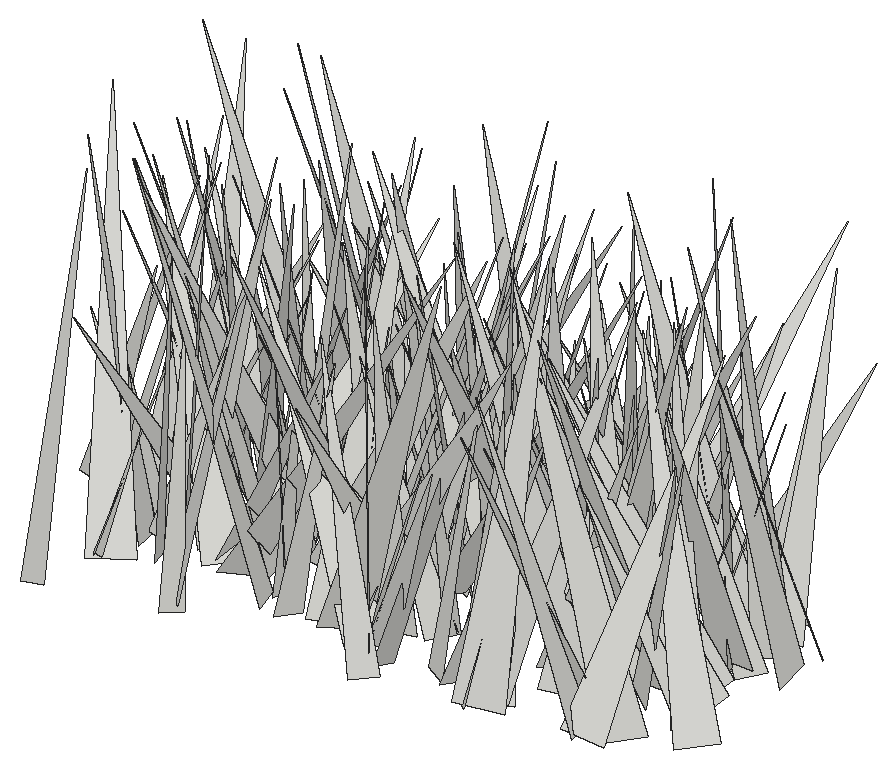
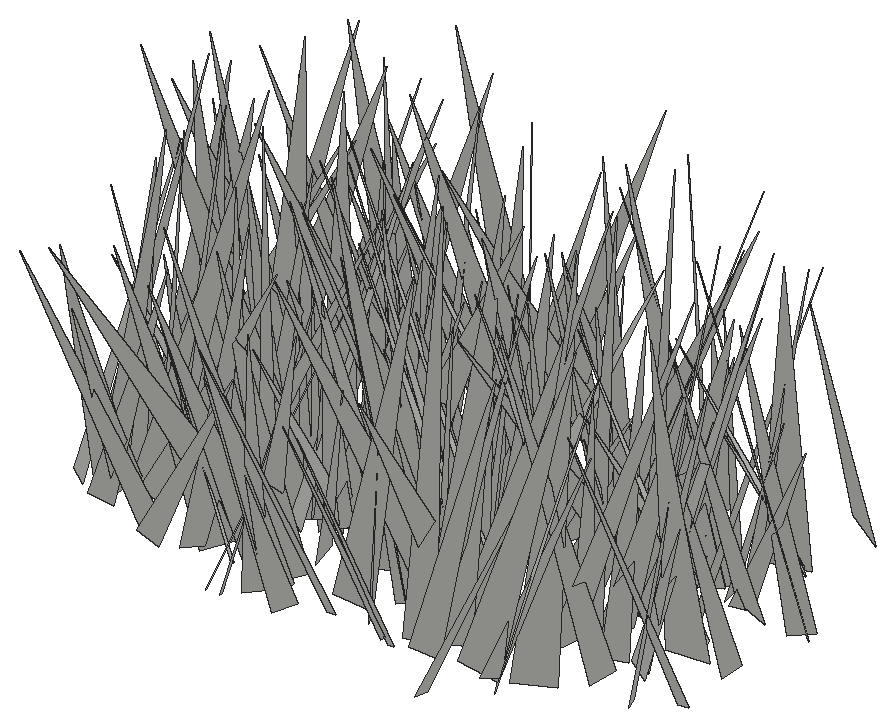
# SketchUp Ruby script. Lengths in inches.
U = 1.inch
M = Sketchup.active_model
def pt(a) = Geom::Point3d.new(a.map { |v| v * U })
def face(e, loops, mat)
  f = e.add_face(loops[0].map { |a| pt(a) })
  loops[1..].each { |l| e.add_face(l.map { |a| pt(a) }).erase! }
  f.material = f.back_material = mat if mat
  f
end
# faces: each face lists its corners as indices into pts; further lists are holes
def faces(e, pts, list, mat = nil) = list.each { |f| face(e, (f[0].is_a?(Array) ? f : [f]).map { |l| l.map { |i| pts[i] } }, mat) }
# xy, xz, yz: faces in a plane at the given z, y or x. An outline is a flat list of corners, or four numbers for a rectangle; further outlines are holes
def ring(l) = l.size == 4 ? [[l[0], l[1]], [l[2], l[1]], [l[2], l[3]], [l[0], l[3]]] : l.each_slice(2).to_a
def flat(e, list, mat, &to3) = list.each { |f| face(e, (f[0].is_a?(Array) ? f : [f]).map { |l| ring(l).map { |u, v| to3.(u, v) } }, mat) }
def xy(e, z, list, mat = nil) = flat(e, list, mat) { |x, y| [x, y, z] }
def xz(e, y, list, mat = nil) = flat(e, list, mat) { |x, z| [x, y, z] }
def yz(e, x, list, mat = nil) = flat(e, list, mat) { |y, z| [x, y, z] }
def lines(e, pts, list) = list.each { |a, b| e.add_line(pt(pts[a]), pt(pts[b])) }
# prism: a flat outline (further loops are holes) pulled along v
def prism(e, loops, v, mat = nil)
  f = face(e, loops, mat); d = Geom::Vector3d.new(v.map { |x| x * U })
  f.pushpull(f.normal.samedirection?(d) ? d.length : -d.length)
end
def box(e, o, s, mat = nil) = prism(e, [[o, [o[0] + s[0], o[1], o[2]], [o[0] + s[0], o[1] + s[1], o[2]], [o[0], o[1] + s[1], o[2]]]], [0, 0, s[2]], mat)
def at(x, y, z, deg = 0) = Geom::Transformation.translation(pt([x, y, z])) * Geom::Transformation.rotation(ORIGIN, Z_AXIS, deg.degrees)
def axes(o, x, y, z) = Geom::Transformation.new([*x, 0, *y, 0, *z, 0, *pt(o).to_a, 1])
def part(name) = M.definitions.add(name)
# library, detail: a bought-in or finely detailed component or shape, given as its bounding box
def library(name, o, s) = part(name).tap { |d| box(d.entities, o, s) }
def detail(e, o, s) = box(e.add_group.entities, o, s)
def put(e, d, t, mat = nil) = e.add_instance(d, t).tap { |i| i.material = mat if mat }
def group(e, t, mat = nil) = e.add_group.tap { |g| g.transformation = t; g.material = mat if mat }.entities
root = M.entities
c1 = part("fur_instance\#9")
p = [[0.8125,0,1.79],[0.67,-0.02,1.48],[0,-0.11,0],[0,0.11,0]]
faces(c1.entities,p,[[0,1,2,3]])
put(root,c1,axes([480.27,96.49,-21.66],[2.16067,6.65454,0.44246],[6.23565,-2.18071,2.34697],[-2.36543,0.32979,6.59114]))
put(root,c1,axes([500.39,100.44,-21.86],[-6.30832,-1.1114,1.05664],[-1.00602,6.37534,0.69964],[1.15742,-0.51611,6.36715]))
put(root,c1,axes([484.89,98.1,-21.86],[-4.63028,1.37895,0.71291],[1.15549,4.55932,-1.31404],[1.03661,1.07721,4.64912]))
put(root,c1,axes([491.26,100.58,-21.66],[3.99613,2.0991,0.80323],[2.24013,-3.58697,-1.77087],[0.18236,-1.93595,4.15203]))
put(root,c1,axes([500.77,100.9,-21.86],[-1.67937,-5.43767,0.87836],[-5.25266,1.30456,-1.96667],[-1.65811,1.37475,5.34049]))
put(root,c1,axes([492.84,98.29,-21.66],[-1.19348,5.65379,0.3473],[5.3271,0.99964,2.033],[-1.92561,-0.73875,5.40894]))
put(root,c1,axes([491.73,100.59,-21.86],[3.13596,-3.23192,0.2957],[-3.22644,-3.06024,0.76944],[0.35051,0.74607,4.43707]))
put(root,c1,axes([490.01,100.77,-21.86],[6.25642,-5.32962,1.03257],[-5.42827,-6.12142,1.29455],[0.06986,1.65444,8.11614]))
put(root,c1,axes([490.73,103.3,-21.86],[5.3138,-2.81187,1.14067],[-1.98861,-4.96443,-2.9739],[-2.29198,-2.2118,5.22484]))
put(root,c1,axes([496.16,99.26,-21.86],[2.60004,3.22909,0.64132],[3.22546,-2.66223,0.32783],[-0.65933,-0.2899,4.13277]))
put(root,c1,axes([490.37,102.97,-21.86],[-0.28332,-7.79704,0.77926],[-7.68212,0.12267,-1.56569],[-1.54472,0.82004,7.64347]))
put(root,c1,axes([491.24,100.57,-21.86],[4.97701,4.02381,2.97396],[4.34378,-5.5566,0.24873],[-2.48337,-1.65505,6.3953]))
put(root,c1,axes([486.82,100.67,-21.86],[-7.32124,-3.15954,0.71739],[-3.23761,7.2018,-1.32279],[0.12329,1.49974,7.86343]))
put(root,c1,axes([487.99,100.38,-21.86],[4.38322,-1.64948,1.59394],[-1.93146,-4.50849,0.64578],[-1.2373,1.19448,4.63858]))
put(root,c1,axes([496.82,99.37,-21.86],[-2.78975,7.45432,2.27613],[7.61508,3.12201,-0.8911],[1.66081,-1.79348,7.90921]))
put(root,c1,axes([497.34,100.01,-21.86],[-1.61358,3.38665,0.61033],[3.4322,1.63258,0.01498],[0.24881,-0.55751,3.75138]))
put(root,c1,axes([481.01,104.5,-21.86],[-5.2943,-3.28141,1.0592],[-2.29433,4.80125,3.40634],[2.57403,-2.46971,5.21479]))
put(root,c1,axes([494.33,100.22,-21.86],[2.52877,4.50107,1.40807],[4.66336,-2.62485,0.01569],[-0.70386,-1.21962,5.16276]))
put(root,c1,axes([494.9375,101.89,-21.86],[3.51068,-4.45404,1.06123],[-4.56743,-3.50052,0.41776],[-0.32136,1.09429,5.65587]))
put(root,c1,axes([491.55,101.67,-21.86],[1.40139,-5.88916,2.09043],[-6.21682,-1.53152,-0.14692],[-0.635,1.99706,6.05182]))
put(root,c1,axes([495.12,100.16,-21.86],[5.00649,-0.69371,1.01239],[-0.92226,-4.93206,1.18126],[-0.80969,1.32843,4.91435]))
put(root,c1,axes([491.03,100.64,-21.86],[-4.99082,4.3261,0.4502],[4.29852,4.80129,1.51542],[-0.66378,-1.43477,6.4286]))
put(root,c1,axes([484.51,98.6,-21.66],[4.61652,6.22378,1.13894],[6.03614,-4.75491,1.51682],[-1.89675,0.0163,7.59914]))
put(root,c1,axes([480.61,99.28,-21.66],[3.00596,2.69315,0.13963],[2.45938,-2.82346,1.51258],[-1.10635,1.04086,3.74179]))
put(root,c1,axes([487.03,101.47,-21.86],[-3.86454,-2.68359,1.87384],[-2.96857,4.09497,-0.25773],[1.3786,1.29506,4.69786]))
put(root,c1,axes([501.93,100.6875,-21.86],[-2.9065,7.574,1.65107],[7.44857,2.24028,2.83534],[-2.14716,-2.4809,7.60092]))
put(root,c1,axes([482.49,101.8,-21.86],[6.26613,3.81902,2.82967],[4.24719,-6.60086,-0.4964],[-2.13385,-1.92357,7.3214]))
put(root,c1,axes([482.27,100.73,-21.86],[-4.86729,-1.78674,2.25978],[-2.35287,5.02555,-1.09424],[1.66225,1.88173,5.06809]))
put(root,c1,axes([486.97,101.35,-21.86],[4.11345,0.18865,1.81103],[0.00918,-4.47631,0.44541],[-1.8208,0.4036,4.09361]))
put(root,c1,axes([481.49,101.72,-21.86],[0.33455,3.97904,1.71347],[4.11253,0.24873,-1.38056],[1.36232,-1.72801,3.74683]))
put(root,c1,axes([489.52,102.44,-21.66],[2.95462,-6.48005,1.02046],[-5.97059,-2.19282,3.36242],[2.71745,2.2277,6.27814]))
put(root,c1,axes([484.28,101.91,-21.86],[4.93305,-2.19664,0.15391],[-2.18894,-4.85066,0.92924],[0.23965,0.9109,5.31946]))
put(root,c1,axes([496.72,100.1875,-21.66],[1.72672,7.47142,1.23195],[7.48463,-1.49226,-1.44043],[1.14896,-1.50745,7.53186]))
put(root,c1,axes([481.16,101.46,-21.86],[-6.73527,-1.87686,1.53677],[-2.12146,6.75676,-1.04577],[1.17629,1.43931,6.91323]))
put(root,c1,axes([500.66,104.12,-21.86],[-0.93689,-7.58778,0.99671],[-7.63501,0.85799,-0.64504],[-0.52389,1.06539,7.61814]))
put(root,c1,axes([481.06,99.66,-21.86],[-3.36629,7.35026,0.38103],[7.33966,3.3212,0.77612],[-0.54849,-0.66835,8.0471]))
put(root,c1,axes([492.88,102.35,-21.86],[-3.29735,3.76242,1.32483],[3.9802,2.99017,1.41439],[-0.2628,-1.92005,4.79874]))
put(root,c1,axes([482,102.76,-21.66],[1.0853,-7.02468,2.48253],[-7.23303,-0.3918,2.05344],[1.78669,2.68091,6.80495]))
put(root,c1,axes([502.95,102.87,-21.86],[-4.62797,0.36048,0.06702],[0.36662,4.56134,0.78248],[0.00509,-0.78533,4.57556]))
put(root,c1,axes([500.76,102.97,-21.66],[-1.89095,-4.65132,2.366],[-4.60338,2.67208,1.57395],[2.45798,1.42605,4.76793]))
put(root,c1,axes([500.77,99.93,-21.86],[-1.75958,6.89289,0.89816],[6.66639,1.93582,-1.79628],[1.96924,-0.39424,6.88342]))
put(root,c1,axes([481.22,102.33,-21.86],[-3.86057,-0.50737,0.50019],[-0.53854,3.88252,-0.21837],[0.46646,0.28336,3.88764]))
put(root,c1,axes([486.08,102.13,-21.66],[-6.99068,-2.50094,0.47101],[-2.54423,6.83653,-1.46112],[-0.05835,1.53405,7.27938]))
put(root,c1,axes([492.55,99.67,-21.86],[7.12647,2.20024,1.82821],[1.44023,-6.99989,2.8102],[-2.47167,2.26505,6.90872]))
put(root,c1,axes([498.96,102.43,-21.86],[-8.06825,0.70999,0.37952],[0.71569,8.07597,0.10667],[0.36866,-0.13964,8.09873]))
put(root,c1,axes([477.54,103.22,-21.66],[1.22983,-5.08709,1.30795],[-5.046,-0.77126,1.74491],[1.45845,1.62123,4.93419]))
put(root,c1,axes([486.28,103.6875,-21.86],[-0.05824,-3.81958,0.55077],[-3.85535,0.08183,0.15984],[0.16986,0.54776,3.81668]))
put(root,c1,axes([485.17,101.18,-21.66],[7.21653,-2.33327,0.39687],[-2.31249,-6.67999,2.77668],[0.50399,2.75925,7.05779]))
put(root,c1,axes([494.375,103.38,-21.86],[7.07527,1.73735,2.55738],[2.12787,-7.36989,-0.88027],[-2.24293,-1.5114,7.23207]))
put(root,c1,axes([483.26,102.41,-21.86],[-3.33055,3.67395,0.98734],[3.8043,3.21801,0.85849],[0.0046,-1.30837,4.884]))
put(root,c1,axes([480.72,99.3,-21.66],[4.07419,5.57288,0.07978],[5.18286,-3.82462,2.48447],[-2.04971,1.40628,6.44076]))
put(root,c1,axes([484.37,101.42,-21.66],[-3.04335,5.85133,0.32291],[5.70958,2.87864,1.64877],[-1.32023,-1.03909,6.38604]))
put(root,c1,axes([480.43,102.84,-21.86],[-2.47066,2.78913,0.64805],[2.82871,2.24449,1.12431],[-0.44456,-1.21919,3.55237]))
put(root,c1,axes([499.96,104.59,-21.66],[5.73315,-1.08828,0.33068],[-0.98004,-5.58896,-1.40205],[-0.57725,-1.3198,5.66459]))
put(root,c1,axes([495.1,102.68,-21.86],[1.88047,-2.78184,1.95652],[-3.20631,-2.19563,-0.04014],[-1.13412,1.59479,3.35756]))
put(root,c1,axes([487.54,103.27,-21.66],[4.40599,-6.63506,1.39046],[-6.52465,-3.70025,3.01783],[1.84021,2.76664,7.37085]))
put(root,c1,axes([504.08,101.87,-21.86],[-4.84886,5.21937,0.60309],[5.25064,4.78392,0.8135],[-0.19034,-0.99462,7.07753]))
put(root,c1,axes([502.84,104.25,-21.86],[-6.49837,1.01991,0.13564],[1.01971,6.26851,1.71854],[-0.13717,-1.71841,6.34946]))
put(root,c1,axes([497.03,103.09,-21.86],[4.67154,-2.82363,0.84685],[-2.94301,-4.55853,1.0353],[-0.16964,1.32674,5.35951]))
put(root,c1,axes([485.5625,104.98,-21.86],[0.24896,-7.3468,1.55373],[-6.97419,-0.80255,-2.67734],[-2.78393,1.35351,6.84612]))
put(root,c1,axes([496.79,105.05,-21.86],[-0.95692,-4.60949,0.0097],[-4.59629,0.95343,-0.35816],[-0.34872,0.08227,4.69412]))
put(root,c1,axes([477.4,103.15,-21.66],[5.01329,4.55618,1.17415],[4.70331,-4.80639,-1.43108],[0.12753,-1.84671,6.62147]))
put(root,c1,axes([481.6,105.86,-21.86],[-5.06426,-4.56399,0.84014],[-4.29824,5.08189,1.69768],[1.74956,-0.72593,6.60262]))
put(root,c1,axes([494.05,106.69,-21.86],[1.8393,-7.94223,0.20343],[-7.82957,-1.84746,-1.33722],[-1.34842,-0.10629,8.04201]))
put(root,c1,axes([482.29,105.44,-21.86],[-3.33298,-6.74445,1.96036],[-6.484,3.7887,2.01069],[2.69971,0.77298,7.24938]))
put(root,c1,axes([491.25,105.73,-21.86],[-3.9717,-6.10655,1.7462],[-5.81347,4.32471,1.90107],[2.55787,0.34722,7.03209]))
put(root,c1,axes([499.71,103.1,-21.86],[-5.36752,5.77658,2.45123],[6.12108,5.53013,0.37117],[1.38195,-2.05828,7.87664]))
put(root,c1,axes([490.59,100.78,-21.66],[4.99959,5.18328,0.38062],[5.01525,-4.9501,1.53324],[-1.36326,0.79826,7.03643]))
put(root,c1,axes([490.82,103.55,-21.86],[-0.11529,-4.79427,2.44231],[-5.06003,0.9271,1.58106],[1.8292,2.26244,4.52754]))
put(root,c1,axes([498.22,101.44,-21.66],[-3.90191,2.21296,0.38649],[1.88444,3.64598,-1.85127],[1.22289,1.44261,4.08594]))
put(root,c1,axes([483.01,105.3125,-21.86],[7.66875,0.29762,1.40281],[0.64374,-7.5341,-1.92071],[-1.28143,-2.00373,7.43029]))
put(root,c1,axes([502.54,104.86,-21.66],[-6.59727,0.97904,0.29915],[1.02311,6.37288,1.70633],[0.03533,-1.73199,6.44755]))
put(root,c1,axes([493.36,102.35,-21.66],[-5.59441,-0.96055,0.72122],[-1.15543,5.24244,-1.98041],[0.32833,2.08191,5.31959]))
put(root,c1,axes([494.81,101.19,-21.86],[3.19327,6.60837,0.52108],[6.51338,-3.23542,1.11669],[-1.23207,0.02336,7.254]))
put(root,c1,axes([487.875,103.87,-21.86],[3.79573,2.84609,1.46317],[3.05532,-3.89817,-0.34352],[-0.95191,-1.16307,4.73179]))
put(root,c1,axes([503.25,102.5,-21.86],[-0.8728,6.82324,1.17968],[6.78553,0.6058,1.51645],[-1.38016,-1.33658,6.7096]))
put(root,c1,axes([501.84,106.55,-21.86],[2.0561,-6.44135,0.2848],[-6.4395,-2.06652,-0.24899],[-0.32395,0.19535,6.75697]))
put(root,c1,axes([498.01,104.34,-21.86],[7.40162,-2.04644,1.37858],[-2.14984,-7.48787,0.42713],[-1.21103,0.78507,7.66743]))
put(root,c1,axes([493.25,106.45,-21.86],[0.94954,-6.1364,0.24208],[-6.03443,-0.88683,1.18943],[1.14,0.41683,6.09444]))
put(root,c1,axes([488.54,104.8,-21.86],[-4.53938,3.59005,2.40826],[4.08452,4.7056,0.68422],[1.41595,-2.06469,5.74685]))
put(root,c1,axes([488.86,104.42,-21.86],[-5.69424,-4.56861,0.52497],[-4.47673,5.31586,-2.29625],[-1.05201,2.10752,6.92992]))
put(root,c1,axes([495.22,106.93,-21.86],[-1.64763,-7.14584,1.34901],[-6.49832,2.06763,3.01567],[3.26416,0.50931,6.68457]))
put(root,c1,axes([494.14,103.96,-21.66],[1.80379,6.11401,2.80003],[6.29213,-2.55743,1.53087],[-2.37284,-2.13386,6.18799]))
put(root,c1,axes([491.125,105.23,-21.86],[-3.66395,-2.75565,0.79106],[-2.79858,3.7164,-0.01609],[0.62239,0.48852,4.58453]))
put(root,c1,axes([486.97,101.8125,-21.66],[3.53249,6.50702,1.2231],[6.07163,-3.73652,2.34297],[-2.64057,0.11331,7.02355]))
put(root,c1,axes([489.43,100.78,-21.86],[-7.03666,4.34174,0.35439],[3.96979,6.66848,-2.87454],[1.79361,2.2741,7.75256]))
put(root,c1,axes([494.19,107,-21.86],[0.44147,-7.17503,0.62576],[-6.54369,-0.13768,3.03788],[3.00878,0.75334,6.51516]))
put(root,c1,axes([487.37,105.11,-21.66],[-2.45268,-3.25533,0.28731],[-3.08329,2.18606,-1.55237],[-1.08306,1.14864,3.76868]))
put(root,c1,axes([495.54,106.64,-21.86],[2.17041,-4.52553,0.56409],[-4.42394,-2.24099,-0.95709],[-1.10786,0.0828,4.92697]))
put(root,c1,axes([482.15,103.04,-21.66],[3.84867,2.11329,0.22175],[1.92609,-3.66331,1.48248],[-0.8974,1.20066,4.13285]))
put(root,c1,axes([482.04,105.78,-21.66],[-2.37076,-5.83706,1.32394],[-5.9146,2.06646,-1.48049],[-0.91737,1.76156,6.12372]))
put(root,c1,axes([498.57,105.28,-21.86],[-5.73495,-0.11109,1.68244],[-0.04447,5.97258,0.24275],[1.68552,-0.22038,5.73089]))
put(root,c1,axes([500.37,104.77,-21.86],[4.86014,-4.74094,2.82615],[-5.30574,-5.05065,0.65171],[-1.52079,2.46963,6.75816]))
put(root,c1,axes([493.5,104.77,-21.86],[-3.65531,3.57205,1.42816],[3.77376,3.712,0.37448],[0.74692,-1.27356,5.09712]))
put(root,c1,axes([494.64,106.42,-21.86],[4.53182,-5.76132,1.66498],[-5.89155,-4.66684,-0.11276],[-1.12014,1.237,7.32923]))
put(root,c1,axes([495.47,107.55,-21.86],[-4.06699,-5.2197,0.56162],[-5.13541,4.10303,0.94539],[1.09007,-0.14467,6.54919]))
put(root,c1,axes([487.62,103.9,-21.86],[-5.55203,-0.57439,2.02149],[-1.15794,5.60149,-1.58866],[1.75372,1.88009,5.3508]))
put(root,c1,axes([491.55,104.43,-21.66],[7.5928,-1.32868,0.07278],[-1.31152,-7.40102,1.71058],[0.22497,1.69728,7.51598]))
put(root,c1,axes([489.6,104.83,-21.86],[-5.21816,-1.76906,1.50642],[-2.07355,5.2165,-1.05669],[1.04846,1.51216,5.4076]))
put(root,c1,axes([496.71,106.64,-21.86],[1.53942,-5.44162,0.89342],[-5.38829,-1.28703,1.44538],[1.17292,1.22946,5.46735]))
put(root,c1,axes([479.99,102.86,-21.86],[1.53889,6.65129,0.3221],[6.53467,-1.57198,1.24039],[-1.28121,-0.02868,6.71336]))
put(root,c1,axes([490.875,107.99,-21.86],[4.29462,-4.11505,0.26594],[-3.98176,-4.23808,-1.27765],[-1.07236,-0.74374,5.80905]))
put(root,c1,axes([482.93,107.72,-21.66],[-1.97553,-6.78705,1.45707],[-6.65434,2.28292,1.61176],[1.97656,0.90224,6.88251]))
put(root,c1,axes([479.74,105.54,-21.86],[5.0651,3.0377,0.15182],[3.00547,-4.95362,-1.15532],[0.46672,-1.0677,5.79207]))
put(root,c1,axes([484.31,103.88,-21.66],[2.91558,3.30379,0.88214],[2.68077,-2.92801,2.10571],[-2.12289,0.83996,3.8706]))
put(root,c1,axes([492.47,106.68,-21.86],[-1.57238,-4.56901,1.11948],[-4.65933,1.35009,-1.0341],[-0.64787,1.37945,4.72005]))
put(root,c1,axes([481.49,108.17,-21.86],[-0.0268,-5.65268,0.22398],[-5.53849,0.07185,1.15049],[1.15241,0.21383,5.53443]))
put(root,c1,axes([495.97,106.74,-21.86],[6.6749,-4.96789,0.00129],[-4.8195,-6.47499,2.02019],[1.20515,1.62135,8.07174]))
put(root,c1,axes([480.45,108.21,-21.86],[-4.17901,-5.88434,0.7845],[-5.89024,4.22956,0.34775],[0.73891,0.43633,7.20893]))
put(root,c1,axes([484.25,103.2,-21.86],[-1.93127,6.17376,0.09606],[5.65668,1.80943,-2.5656],[2.47519,0.68189,5.93825]))
put(root,c1,axes([493.01,105.88,-21.66],[-4.31341,6.46311,1.11663],[6.32564,3.74609,2.75266],[-1.73345,-2.41229,7.26637]))
put(root,c1,axes([488.35,106.6,-21.86],[3.07396,-3.53335,0.83024],[-3.61315,-2.87553,1.13994],[0.34489,1.36741,4.5425]))
put(root,c1,axes([502.53,106.66,-21.86],[-2.9134,4.03937,1.46912],[4.26943,2.51447,1.5531],[-0.49677,-2.07934,4.73205]))
put(root,c1,axes([486.91,107.17,-21.86],[7.11507,4.33314,0.48127],[4.20256,-6.57141,-2.9643],[1.16029,-2.76992,7.78545]))
put(root,c1,axes([490.875,104.99,-21.66],[4.03542,0.28371,1.50858],[-0.2798,-4.0361,1.5075],[-1.50932,1.50677,3.754]))
put(root,c1,axes([477.96,106.37,-21.86],[4.29201,-0.29938,0.77765],[-0.39482,-4.32378,0.51456],[-0.73381,0.57535,4.27156]))
put(root,c1,axes([499.73,105.29,-21.66],[-6.28866,-0.36775,1.68536],[-0.82762,6.23312,-1.72806],[1.51351,1.8804,6.05775]))
put(root,c1,axes([503.61,107.47,-21.86],[-7.78363,-1.77881,1.5879],[-1.77027,7.9428,0.22014],[1.59741,0.13482,7.98126]))
put(root,c1,axes([482.75,106.56,-21.86],[-5.38349,2.8617,0.60302],[2.91403,5.35589,0.59819],[0.24775,-0.81245,6.06741]))
put(root,c1,axes([500.29,107.11,-21.86],[4.56554,2.4835,0.72557],[2.58092,-4.47494,-0.92307],[-0.18188,-1.15993,5.11467]))
put(root,c1,axes([479.25,110.09,-21.86],[-6.01376,-4.74049,2.00405],[-3.98095,6.23797,2.80955],[3.26197,-1.12665,7.12348]))
put(root,c1,axes([488.32,106.99,-21.86],[1.74245,-3.02379,2.07472],[-3.3962,-2.19711,-0.34987],[-1.38332,1.58534,3.47232]))
put(root,c1,axes([490.18,107.47,-21.86],[-0.07815,-6.05054,2.52953],[-6.4447,0.53908,1.09033],[1.2138,2.47266,5.952]))
put(root,c1,axes([494.47,106.49,-21.86],[-3.32764,3.062,1.30373],[3.08153,3.53122,-0.42827],[1.25687,-0.55083,4.50173]))
put(root,c1,axes([485.02,106.39,-21.86],[4.79862,3.05458,1.6678],[3.017,-5.06719,0.60002],[-1.73486,-0.36311,5.65661]))
put(root,c1,axes([496.94,107.87,-21.86],[-2.89308,-3.13599,0.85003],[-3.23039,2.89836,-0.3018],[0.34876,0.83187,4.25597]))
put(root,c1,axes([500.62,104.97,-21.86],[4.22042,3.02936,0.44277],[2.70703,-4.0447,1.87014],[-1.43005,1.2839,4.84681]))
put(root,c1,axes([497.52,108.96,-21.86],[-6.50951,0.22142,0.60358],[0.38251,6.26967,1.82536],[0.51674,-1.85181,6.25226]))
put(root,c1,axes([485.5,105.07,-21.86],[5.52585,4.05046,1.31825],[3.69086,-5.63091,1.83015],[-2.12639,0.75214,6.60241]))
put(root,c1,axes([489.25,108.11,-21.86],[2.58883,2.26123,2.35644],[2.87323,-3.00647,-0.27159],[-1.55259,-1.79333,3.42658]))
put(root,c1,axes([491.08,105.37,-21.86],[3.08355,6.47581,0.56476],[6.50039,-3.07095,-0.27862],[0.00972,-0.62967,7.16706]))
put(root,c1,axes([489.83,105.62,-21.86],[6.38887,5.18246,1.59043],[5.07791,-6.58181,1.04866],[-1.89794,-0.16426,8.1594]))
put(root,c1,axes([503.1,109.5,-21.86],[-3.86726,-4.8383,0.71579],[-4.78645,3.93151,0.71436],[1.00566,0.10641,6.1526]))
put(root,c1,axes([502.23,108.01,-21.86],[1.93856,-5.12728,2.24723],[-5.46022,-2.25638,-0.43794],[-1.23493,1.9279,5.46399]))
put(root,c1,axes([499.76,108.83,-21.86],[4.54557,4.08977,3.87164],[5.12111,-5.0718,-0.65499],[-2.34307,-3.15097,6.07942]))
put(root,c1,axes([491.375,107.35,-21.86],[6.39922,1.66084,0.77373],[1.68967,-6.43637,-0.15871],[-0.70856,-0.34898,6.60932]))
put(root,c1,axes([480.73,107.49,-21.86],[2.96491,4.33641,3.25393],[4.46173,-4.05854,1.34327],[-3.07985,-1.70497,5.07846]))
put(root,c1,axes([486.71,109.41,-21.86],[-4.58981,-6.81856,1.14154],[-6.9132,4.53833,-0.68805],[0.05895,1.33156,8.19058]))
put(root,c1,axes([484.09,106.55,-21.86],[1.02305,5.31057,1.33507],[5.15193,-1.39366,1.59576],[-1.8553,-0.94167,5.16743]))
put(root,c1,axes([500.87,108.34,-21.86],[-7.81883,2.51294,1.68172],[2.76611,7.82758,1.16397],[1.22135,-1.64052,8.12983]))
put(root,c1,axes([488.61,109.1,-21.86],[-2.51428,-3.3921,0.48717],[-3.39486,2.54791,0.21985],[0.4675,0.25907,4.21659]))
put(root,c1,axes([486.87,108.37,-21.86],[6.0574,2.72005,0.2303],[2.69232,-5.86042,-1.5971],[0.45071,-1.54939,6.44516]))
put(root,c1,axes([497.93,109.04,-21.66],[1.41621,-4.16021,0.5332],[-4.01988,-1.18575,1.42542],[1.19673,0.94019,4.15706]))
put(root,c1,axes([486.52,110.77,-21.86],[5.05065,-5.78899,0.88016],[-5.66798,-5.12516,-1.18448],[-1.47008,-0.1285,7.59069]))
put(root,c1,axes([488.78,108.4375,-21.86],[4.08139,-3.20586,0.61223],[-3.2526,-3.91407,1.18774],[0.27008,1.30866,5.05219]))
put(root,c1,axes([479.77,106.4375,-21.86],[-1.40207,7.22786,1.13046],[7.31414,1.36087,0.37039],[-0.15287,-1.17973,7.35327]))
put(root,c1,axes([501.89,106.46,-21.66],[-7.32928,-2.99407,2.48715],[-3.76161,6.81126,-2.88543],[1.00033,3.67572,7.37273]))
put(root,c1,axes([489.03,109.25,-21.86],[1.53835,-7.01276,2.03333],[-7.04829,-0.88366,2.28484],[1.90652,2.39168,6.80623]))
put(root,c1,axes([488.04,109.26,-21.86],[-2.86919,-3.90872,1.79506],[-4.01549,3.2075,0.56601],[1.54149,1.08002,4.8156]))
put(root,c1,axes([482.52,111.15,-21.86],[4.1786,-6.03386,0.40804],[-6.0035,-4.19846,-0.60465],[-0.72937,-0.01047,7.31455]))
put(root,c1,axes([483.4,108.6,-21.86],[-8.2127,0.65784,0.53458],[0.66874,8.22786,0.14871],[0.52088,-0.19122,8.23766]))
put(root,c1,axes([494.93,109.64,-21.86],[7.08469,1.17747,2.52447],[1.61288,-7.35894,-1.094],[-2.27113,-1.55299,7.09806]))
put(root,c1,axes([483.45,110.95,-21.86],[-2.96228,-3.48582,0.87467],[-2.85625,2.97145,2.16874],[2.18125,-0.843,4.02773]))
put(root,c1,axes([494.78,109.41,-21.86],[3.92592,-0.41216,0.89749],[-0.2951,-4.00034,-0.54626],[-0.94248,-0.46433,3.90952]))
put(root,c1,axes([502.49,108.37,-21.86],[1.97558,6.78512,3.04566],[6.89111,-2.85534,1.89119],[-2.79761,-2.24188,6.80913]))
put(root,c1,axes([494.43,106.28,-21.86],[4.15865,3.49208,0.81847],[2.77358,-3.92559,2.6563],[-2.27416,1.59814,4.73636]))
put(root,c1,axes([487.29,111.21,-21.86],[-0.53699,-7.34105,1.16615],[-7.27133,0.76139,1.44476],[1.5423,1.0337,7.21748]))
put(root,c1,axes([486.96,110.8,-21.66],[-5.96376,-1.66281,1.60864],[-1.32131,6.09893,1.40577],[1.89916,-0.97833,6.02952]))
put(root,c1,axes([481.04,109.34,-21.86],[6.32916,0.13104,0.27334],[0.13733,-6.3333,-0.14369],[-0.27023,-0.14945,6.32889]))
put(root,c1,axes([500.0625,109.18,-21.86],[-2.44299,5.49091,1.30941],[5.27932,1.71736,2.64808],[-1.99837,-2.17564,5.395]))
put(root,c1,axes([501.52,110.27,-21.86],[0.38107,-4.3176,1.24457],[-4.35966,-0.65774,-0.94692],[-1.08815,1.12319,4.22969]))
put(root,c1,axes([477.57,109.43,-21.66],[2.82226,4.09729,0.68802],[3.94816,-2.38599,-1.98631],[1.29353,-1.65697,4.56152]))
put(root,c1,axes([493.41,108.64,-21.86],[-4.4304,-0.23548,0.66281],[-0.42328,4.26855,-1.31284],[0.56178,1.35914,4.23796]))
put(root,c1,axes([493.29,110.49,-21.86],[4.31446,-3.71791,0.40504],[-3.72385,-4.21342,0.9907],[0.3462,1.01276,5.60856]))
put(root,c1,axes([489.88,108.81,-21.86],[-4.49953,-3.59508,3.80394],[-4.60675,5.10137,-0.62788],[2.48443,2.94818,5.72505]))
put(root,c1,axes([497.02,110.74,-21.86],[4.62611,-3.05223,2.53258],[-2.97331,-5.24406,-0.88892],[-2.62479,0.5609,5.47054]))
put(root,c1,axes([495.26,111.16,-21.66],[3.7363,2.07589,0.22504],[1.88074,-3.14536,-2.2112],[0.90706,-2.02911,3.65784]))
put(root,c1,axes([495,109.91,-21.86],[1.4221,-3.78822,2.5832],[-4.25079,-2.10312,-0.74405],[-1.71882,2.06693,3.97736]))
put(root,c1,axes([495.14,112.58,-21.86],[-4.66281,-2.88259,0.04543],[-2.761,4.48988,1.50703],[0.82963,-1.25893,5.27068]))
put(root,c1,axes([483.75,111.94,-21.66],[-4.12735,0.23871,1.0618],[0.66209,3.85593,1.70672],[0.86374,-1.81501,3.76552]))
put(root,c1,axes([487.08,109.51,-21.86],[6.3813,-2.25892,0.20905],[-2.20352,-6.02357,2.17449],[0.53935,2.11689,6.41056]))
put(root,c1,axes([494.68,110.34,-21.86],[3.58397,-3.64133,0.7361],[-3.60405,-3.15993,1.91614],[0.90107,1.84433,4.7363]))
put(root,c1,axes([486.7,111.71,-21.86],[0.91416,-4.94391,1.27953],[-4.9749,-1.15567,-0.91103],[-1.1532,1.06645,4.94449]))
put(root,c1,axes([494.43,112.81,-21.86],[-3.17214,-2.54983,0.51656],[-2.07776,2.97317,1.9168],[1.56569,-1.22048,3.59026]))
put(root,c1,axes([489.6,110.9375,-21.86],[2.96101,1.91002,1.7712],[2.18546,-3.28075,-0.11568],[-1.41742,-1.06838,3.5217]))
put(root,c1,axes([496.55,110.29,-21.86],[3.63193,-4.05591,1.60644],[-4.34601,-3.18259,1.79036],[0.37856,2.37544,5.14159]))
put(root,c1,axes([490.44,110.81,-21.66],[0.55965,-6.1533,3.26603],[-6.71098,-1.35523,-1.40332],[-1.86889,3.02383,6.01722]))
put(root,c1,axes([487.91,108.15,-21.86],[-4.47907,3.89554,0.463],[3.44419,4.24137,-2.36643],[1.87807,1.51235,5.44401]))
put(root,c1,axes([502.29,108.7,-21.66],[-5.42402,3.35952,0.54018],[3.08821,5.28712,-1.87283],[1.42868,1.32596,6.09909]))
put(root,c1,axes([501.15,109.28,-21.66],[-4.3486,2.21974,0.80785],[1.83051,4.23636,-1.78683],[1.49303,1.27131,4.54366]))
put(root,c1,axes([488.36,111.75,-21.86],[2.45066,3.05169,0.44917],[2.65928,-1.79957,-2.28257],[1.56295,-1.7231,3.17938]))
put(root,c1,axes([493.63,111.9,-21.86],[3.58428,-2.61771,1.24135],[-2.70899,-3.7283,-0.04015],[-1.02701,0.69843,4.43823]))
put(root,c1,axes([484.53,111.57,-21.86],[0.18988,-6.4583,3.19895],[-6.79344,-1.22898,-2.07794],[-2.40669,2.95955,6.11783]))
put(root,c1,axes([498.61,111.09,-21.66],[0.87918,5.14411,1.43079],[4.85097,-0.16366,-2.39235],[2.23095,-1.67133,4.63805]))
put(root,c1,axes([498.44,111.66,-21.66],[-0.27177,-3.75184,1.87256],[-3.70908,-0.66019,-1.86105],[-1.95589,1.77327,3.26904]))
put(root,c1,axes([483.75,111.48,-21.86],[-6.3033,-3.29184,1.05702],[-3.45211,6.11366,-1.54635],[0.19083,1.86335,6.94094]))
put(root,c1,axes([492.19,112.23,-21.86],[3.34433,-2.45993,0.06359],[-2.39384,-3.22746,1.0454],[0.56992,0.87868,4.01783]))
put(root,c1,axes([492.83,111.53,-21.86],[6.76067,1.19839,0.69108],[1.18973,-6.79585,0.14582],[-0.7059,0.02372,6.86451]))
put(root,c1,axes([487.88,112.01,-21.86],[2.51119,2.94201,0.30611],[2.79372,-2.22715,-1.51331],[0.97173,-1.19981,3.55969]))
put(root,c1,axes([496.4375,108.93,-21.66],[-2.65177,6.66161,0.65253],[5.97681,2.67255,-2.995],[3.01341,0.56142,6.51452]))
put(root,c1,axes([490.56,111.8125,-21.66],[2.95433,4.07724,0.35212],[3.82019,-2.59183,-2.04072],[1.46767,-1.46099,4.60298]))
put(root,c1,axes([485.03,113.9375,-21.86],[-4.59731,-1.23154,0.33008],[-1.08177,4.4213,1.42926],[0.67485,-1.30242,4.53973]))
